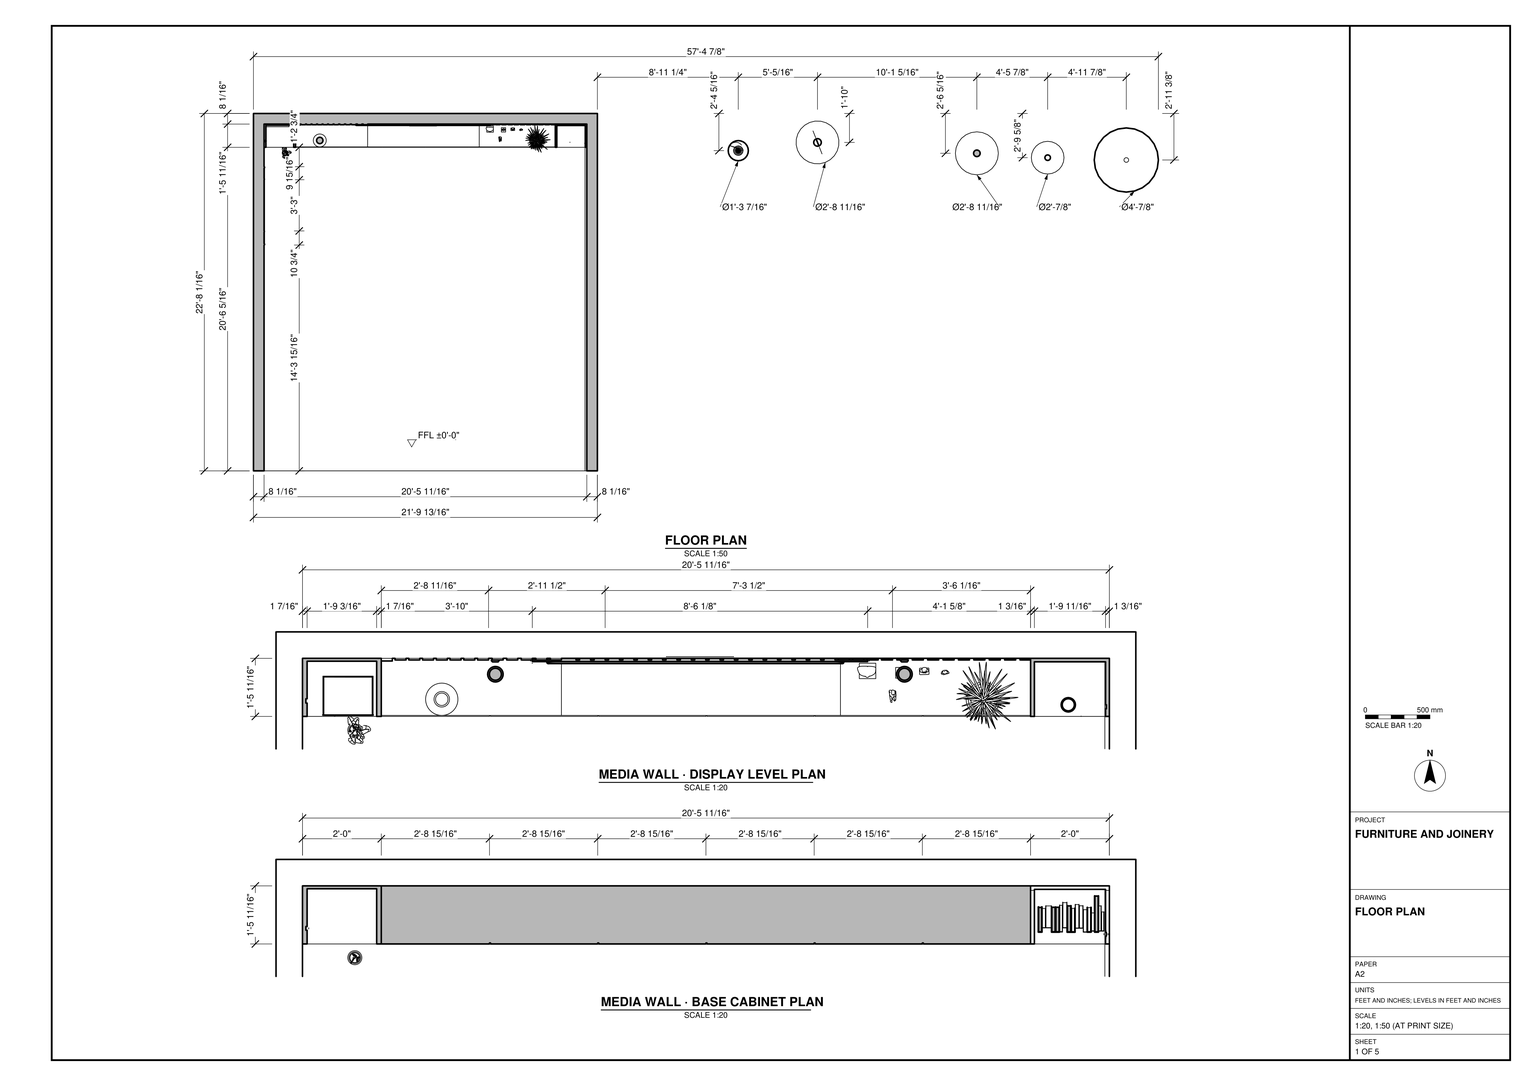
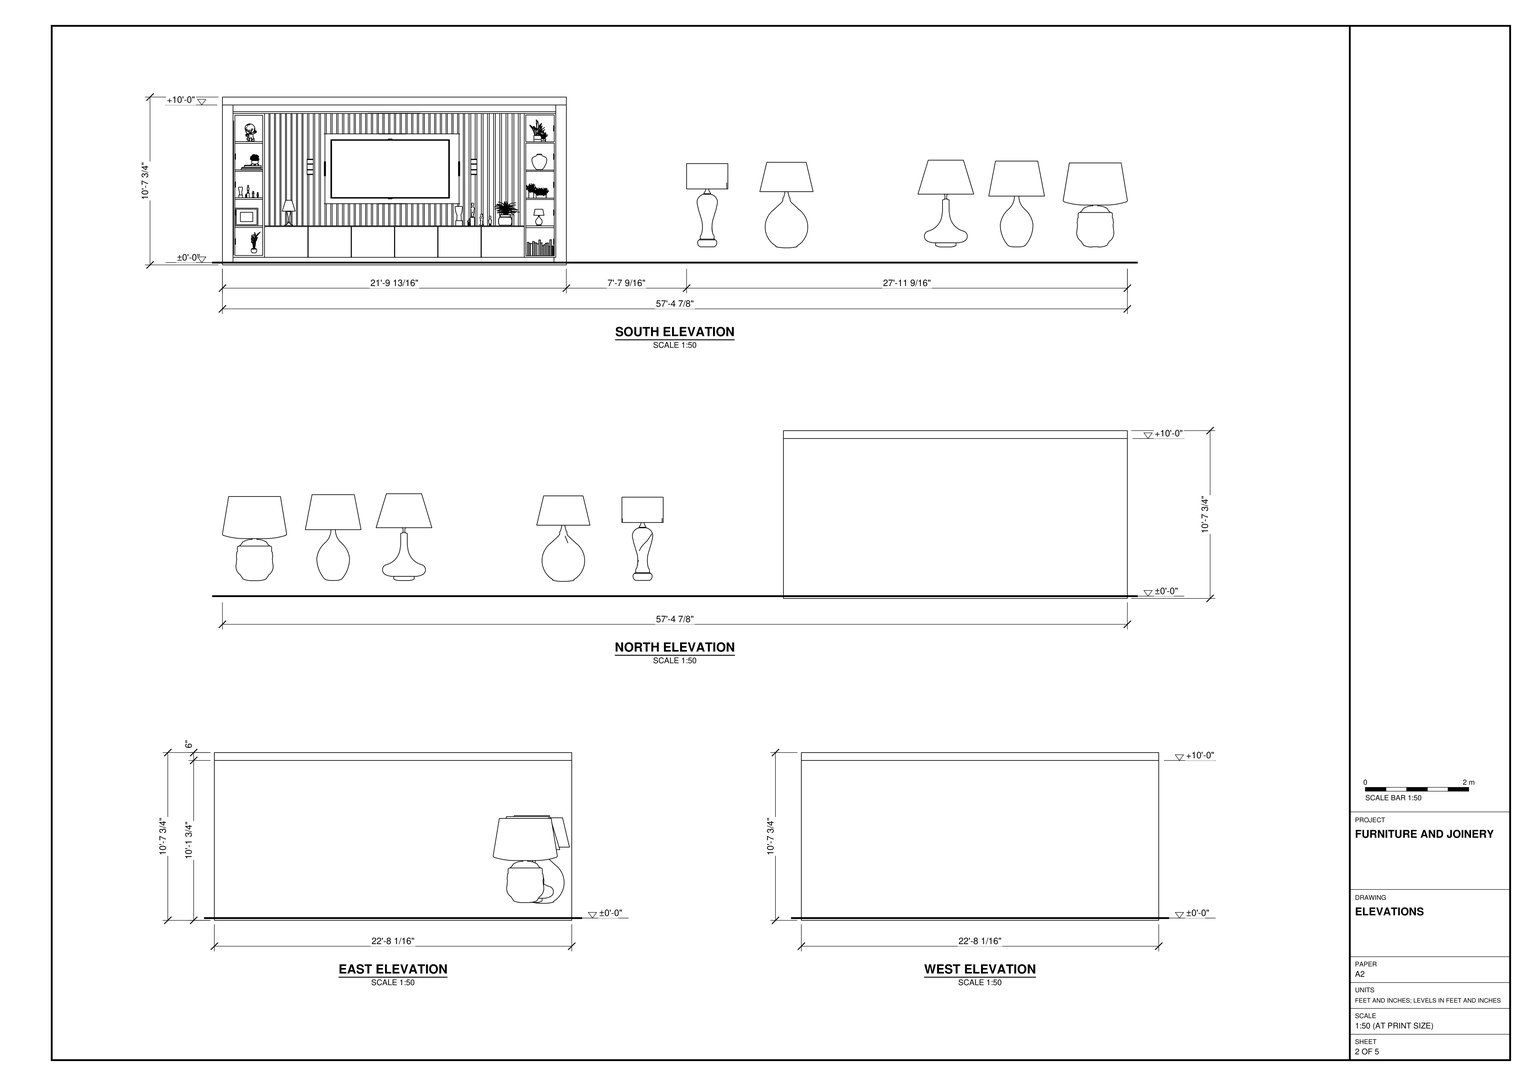
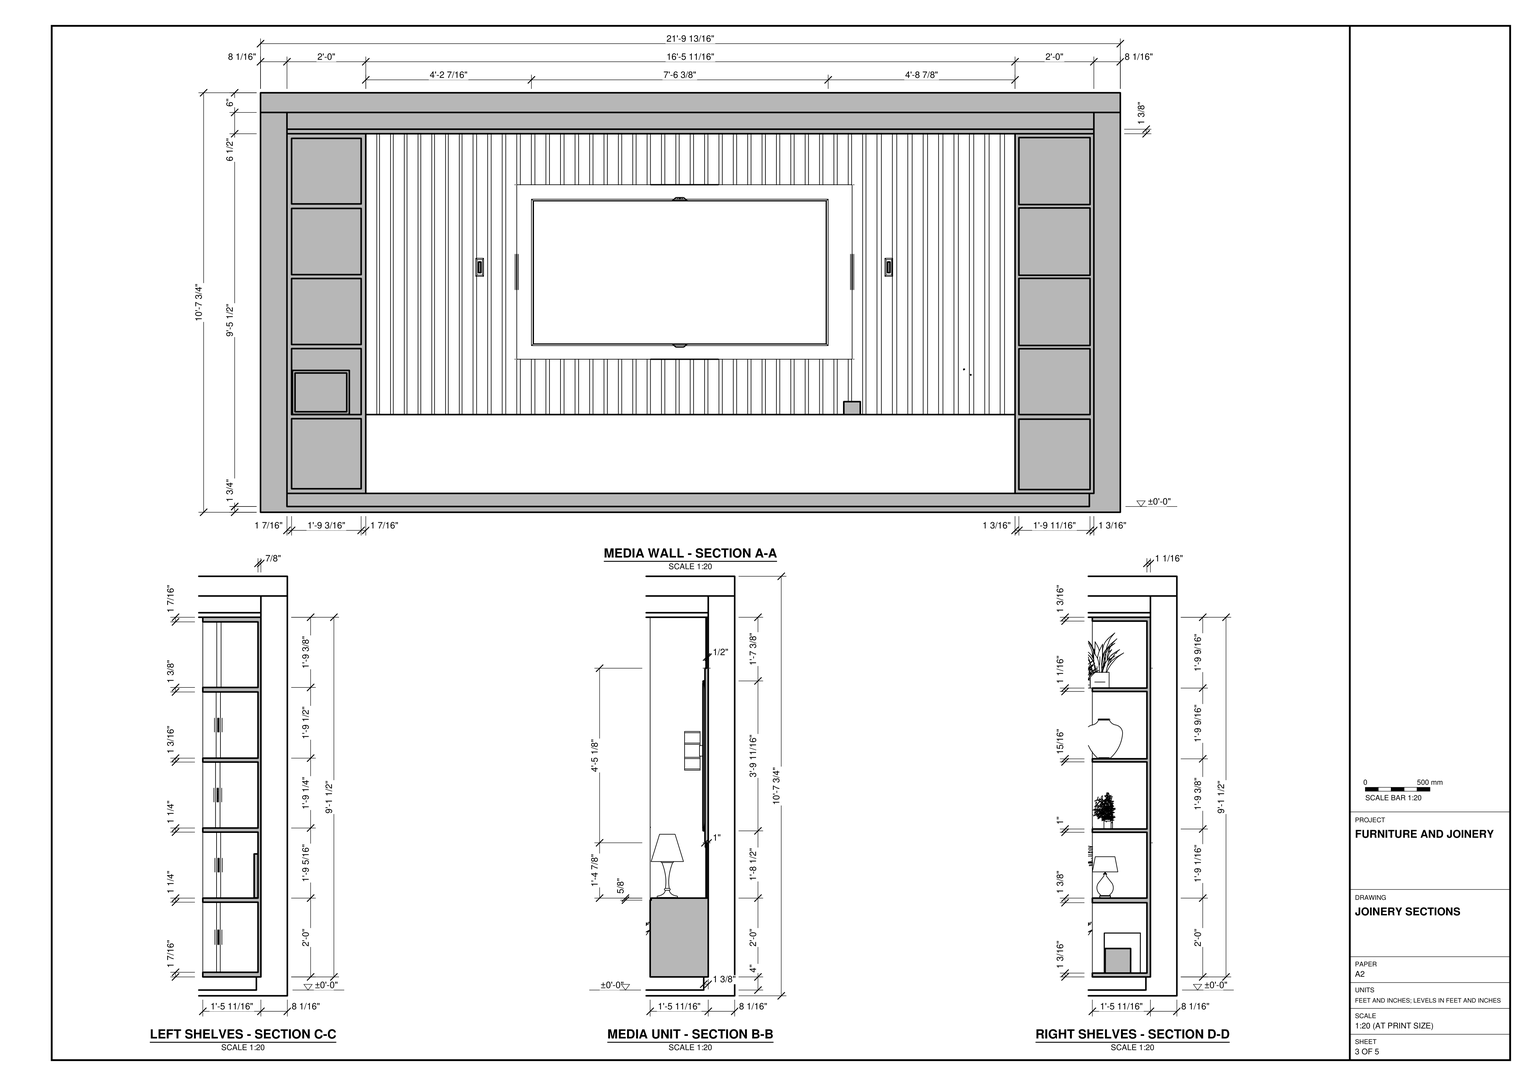
Model the media wall and its three-sided room shell in SketchUp from task_files/diagram_01.pdf. Work in feet and inches, with the finished floor at ±0'-0". Including the freestanding lamps to the right of the shell, the overall model is 57'-4 7/8" wide, 22'-8 1/16" deep and 10'-7 3/4" high. Use the 8 1/16" wall thickness shown in plan. Include the floor slab, upper slab and window unit, and leave the front open as shown in the south elevation.

Fit the joinery across the 20'-5 11/16" clear width of the rear wall. Use the base cabinet plan to divide the low cabinet run into six equal fronts above a recessed plinth. At each end, build a tall open shelving unit with the shelf spacing shown in its section. Between the shelving units, model the vertical slats behind the framed rectangular display. Place the books, plants and small display objects on the shelves and cabinet top. Position the five freestanding lamps as shown in plan, preserving the larger gap between the second and third lamps. Any suitable library components may be used for lamps, plants, books and other loose items.

Keep each shell element and each furniture or joinery piece in a separate group or component, and use components for repeated parts. Save one SketchUp model as output_files/built_in_media_wall_with_flanking_display_shelves.skp.

# SketchUp Ruby script. Lengths in inches.
U = 1.inch
M = Sketchup.active_model
def pt(a) = Geom::Point3d.new(a.map { |v| v * U })
def face(e, loops, mat)
  f = e.add_face(loops[0].map { |a| pt(a) })
  loops[1..].each { |l| e.add_face(l.map { |a| pt(a) }).erase! }
  f.material = f.back_material = mat if mat
  f
end
# faces: each face lists its corners as indices into pts; further lists are holes
def faces(e, pts, list, mat = nil) = list.each { |f| face(e, (f[0].is_a?(Array) ? f : [f]).map { |l| l.map { |i| pts[i] } }, mat) }
# xy, xz, yz: faces in a plane at the given z, y or x. An outline is a flat list of corners, or four numbers for a rectangle; further outlines are holes
def ring(l) = l.size == 4 ? [[l[0], l[1]], [l[2], l[1]], [l[2], l[3]], [l[0], l[3]]] : l.each_slice(2).to_a
def flat(e, list, mat, &to3) = list.each { |f| face(e, (f[0].is_a?(Array) ? f : [f]).map { |l| ring(l).map { |u, v| to3.(u, v) } }, mat) }
def xy(e, z, list, mat = nil) = flat(e, list, mat) { |x, y| [x, y, z] }
def xz(e, y, list, mat = nil) = flat(e, list, mat) { |x, z| [x, y, z] }
def yz(e, x, list, mat = nil) = flat(e, list, mat) { |y, z| [x, y, z] }
def lines(e, pts, list) = list.each { |a, b| e.add_line(pt(pts[a]), pt(pts[b])) }
# prism: a flat outline (further loops are holes) pulled along v
def prism(e, loops, v, mat = nil)
  f = face(e, loops, mat); d = Geom::Vector3d.new(v.map { |x| x * U })
  f.pushpull(f.normal.samedirection?(d) ? d.length : -d.length)
end
def box(e, o, s, mat = nil) = prism(e, [[o, [o[0] + s[0], o[1], o[2]], [o[0] + s[0], o[1] + s[1], o[2]], [o[0], o[1] + s[1], o[2]]]], [0, 0, s[2]], mat)
def at(x, y, z, deg = 0) = Geom::Transformation.translation(pt([x, y, z])) * Geom::Transformation.rotation(ORIGIN, Z_AXIS, deg.degrees)
def axes(o, x, y, z) = Geom::Transformation.new([*x, 0, *y, 0, *z, 0, *pt(o).to_a, 1])
def part(name) = M.definitions.add(name)
# library, detail: a bought-in or finely detailed component or shape, given as its bounding box
def library(name, o, s) = part(name).tap { |d| box(d.entities, o, s) }
def detail(e, o, s) = box(e.add_group.entities, o, s)
def put(e, d, t, mat = nil) = e.add_instance(d, t).tap { |i| i.material = mat if mat }
def group(e, t, mat = nil) = e.add_group.tap { |g| g.transformation = t; g.material = mat if mat }.entities
root = M.entities
M.materials.add("Generic").color = [230, 212, 196]
M.materials.add("[Color C01]").color = [255, 229, 204]
M.materials.add("[Color D01]").color = [168, 159, 134]
M.materials.add("[Color M08]").color = [30, 30, 30]
M.materials.add("[Color_008]").color = [30, 30, 30]
M.materials.add("[Granite Dark Gray]").color = [69, 68, 68]
M.materials.add("[Groundcover_RiverRock_4inch]").color = [145, 126, 109]
c1 = library("Wall+spot",[0,0,0],[4.72,6.7,11.8125])
c2 = library("Flat screen television",[0,1.41,1.14],[35.92,0.28,20.21])
c3 = library("Spot Light",[-5.1,-5.1,-11.05],[10.2,10.2,11.05])
c4 = library("Spot Light\#1",[-5.1,-5.1,-11.05],[10.2,10.2,11.05])
c5 = library("ADORNOS+LIVROS+PLANTA+CELULAR+ÓCULOS",[6.19,-1.3125,-0.22],[15.35,11.9,12.07])
c6 = library("Cycladic+Idols",[-6.2,-43.67,0],[139.39,59.86,86.49])
c7 = part("Picture frame")
xy(c7.entities,0,[[[-0.79,-0.79,16.54,12.6],[0,0,15.75,11.8125]],[[0,0,15.75,11.8125],[3.15,2.36,12.6,9.45]]])
xy(c7.entities,0.79,[[[0,0,15.75,11.8125],[3.15,2.36,12.6,9.45]]])
xy(c7.entities,1.18,[[[-0.79,-0.79,16.54,12.6],[0,0,15.75,11.8125]]],"[Color_008]")
xz(c7.entities,-0.79,[[-0.79,0,16.54,1.18]],"[Color_008]")
xz(c7.entities,0,[[0,0,15.75,0.79]])
xz(c7.entities,0,[[0,0.79,15.75,1.18]],"[Color_008]")
xz(c7.entities,2.36,[[3.15,0,12.6,0.79]])
xz(c7.entities,9.45,[[3.15,0,12.6,0.79]])
xz(c7.entities,11.8125,[[0,0,15.75,0.79]])
xz(c7.entities,11.8125,[[0,0.79,15.75,1.18]],"[Color_008]")
xz(c7.entities,12.6,[[-0.79,0,16.54,1.18]],"[Color_008]")
yz(c7.entities,-0.79,[[-0.79,0,12.6,1.18]],"[Color_008]")
yz(c7.entities,0,[[0,0,11.8125,0.79]])
yz(c7.entities,0,[[0,0.79,11.8125,1.18]],"[Color_008]")
yz(c7.entities,3.15,[[2.36,0,9.45,0.79]])
yz(c7.entities,12.6,[[2.36,0,9.45,0.79]])
yz(c7.entities,15.75,[[0,0,11.8125,0.79]])
yz(c7.entities,15.75,[[0,0.79,11.8125,1.18]],"[Color_008]")
yz(c7.entities,16.54,[[-0.79,0,12.6,1.18]],"[Color_008]")
g1 = group(c7.entities,at(0,0,0.79))
xy(g1,0,[[3.15,2.36,12.6,9.45]],"[Groundcover_RiverRock_4inch]")
c8 = library("Potted broadleaf plant",[-29.7,0,-10.87],[31.67,38.52,72.45])
c9 = library("Potted plant pair",[-0.125,-0.11,0],[4.84,5.4,5.74])
c10 = library("interior plants_leaves_small",[-1.83,-3.05,0],[40.47,20.87,24.79])
c11 = library("Pot+Nice",[-24.73,-24.73,-0.79],[49.46,49.46,53.07])
c12 = library("Architecture and design books\#1",[9.67,-0.02,0],[20.02,11.1,12.25])
c13 = library("Potted+Plant",[38.42,1.35,0],[44.68,49.99,41.74])
c14 = library("lamp",[0,0,0],[9.82,9.84,19.44])
c15 = library("Mesh Light\#5",[-0.5,-0.5,-0.1],[1,1,0.2])
c16 = library("Group\#3",[-0.5,-0.5,0],[1,1.5,53.15])
c17 = library("Group\#4",[-0.5,-0.5,-0.1],[103.125,2,0.2])
c18 = library("Group\#5",[-0.5,-0.5,0],[1,1.5,53.15])
c19 = library("Group\#6",[-0.5,-0.5,-0.1],[103.125,2,0.2])
c20 = library("Group\#9",[-0.5,-0.5,0],[1.375,2.125,21.34])
c21 = library("Group\#10",[-0.5,-0.5,0],[1.375,2.25,20.09])
c22 = library("Group\#11",[-0.5,-0.5,0],[1.375,2.375,20.09])
c23 = library("Group\#13",[-0.5,-0.5,0],[1.375,2.3125,20.15])
c24 = library("Group\#17",[-0.5,-0.5,0],[1.25,2.1875,21.4375])
c25 = library("Group\#18",[-0.5,-0.5,0],[1.25,2,20.04])
c26 = library("Group\#19",[-0.5,-0.5,0],[1.25,2,20.4375])
c27 = library("Group\#21",[-0.5,-0.5,0],[1.25,3.07,41.9375])
c28 = library("Group\#26",[0,0,0],[2.77,2.73,4.26])
c29 = library("Group\#40",[0,0,0],[31.4,31.4,63.39])
c30 = library("Group\#39",[0,0,0],[67.07,67.07,107.62])
c31 = library("Group\#38",[0,0,0],[83.73,83.73,135.9375])
c32 = library("Group\#37",[0,0,0],[48.82,48.82,75.96])
c33 = library("Group\#36",[0,0,0],[51.75,51.75,79.68])
c34 = library("Group\#35",[0,0,0],[64.77,64.77,84.93])
xy(root,0,[[0,0,261.8125,272.0625]])
xy(root,1.75,[[8.05,0,252.38,262.63]],"Generic")
xy(root,5.75,[[252.38,0,253.76,246.32],[8.05,246.32,32.05,262.63],[32.05,246.32,32.05,262.63,229.76,262.63,229.76,246.32,197.11,246.32,197.11,246.62,196.81,246.62,196.81,246.32,164.16,246.32,164.16,246.62,163.86,246.62,163.86,246.32,131.21,246.32,131.21,246.62,130.91,246.62,130.91,246.32,98.26,246.32,98.26,246.62,97.96,246.62,97.96,246.32,65.3,246.32,65.3,246.62,65,246.62,65,246.32],[229.76,246.32,252.38,262.63],[252.38,246.32,253.76,262.63],
  [8.05,262.63,32.05,264.01],[32.05,262.63,229.76,264.01],[229.76,262.63,253.76,264.01]])
xy(root,6.92,[[252.38,246.32,252.59,246.32,252.59,248.7,252.84,248.7,252.84,249.88,252.59,249.88,252.59,262.95,252.38,262.95]])
xy(root,6.92,[[230.93,246.32,252.38,262.95]],"[Color C01]")
xy(root,7.16,[[9.46,246.32,30.64,246.32,30.64,263.13,9.46,263.13,9.46,251.63,9.09,251.63,9.09,250.51,9.46,250.51]],"[Color C01]")
xy(root,28.36,[[252.38,246.32,252.38,262.95,252.59,262.95,252.59,249.88,252.84,249.88,252.84,248.7,252.59,248.7,252.59,246.32]])
xy(root,28.36,[[230.93,246.32,252.38,262.95]],"[Color C01]")
xy(root,28.5,[[9.46,246.32,9.46,250.51,9.09,250.51,9.09,251.63,9.46,251.63,9.46,263.13,30.64,263.13,30.64,246.32]],"[Color C01]")
xy(root,29.125,[[32.05,246.32,65,246.62],[65.3,246.32,97.96,246.62],[98.26,246.32,130.91,246.62],[131.21,246.32,163.86,246.62],[164.16,246.32,196.81,246.62],
  [197.11,246.32,229.76,246.62]])
xy(root,29.75,[[9.46,246.32,30.64,246.32,30.64,263.13,9.46,263.13,9.46,251.76,9.09,251.76,9.09,250.51,9.46,250.51],[252.38,246.32,252.59,246.32,252.59,248.88,252.84,248.88,252.84,249.88,252.59,249.88,252.59,262.95,252.38,262.95],[32.05,263.2,35.4,264.01],[36.24,263.51,39.59,264.01],[40.43,263.51,43.78,264.01],
  [44.62,263.51,47.97,264.01],[48.8,263.51,52.15,264.01],[52.99,263.51,56.34,264.01],[57.18,263.51,60.53,264.01],[61.37,263.51,64.72,264.01],
  [65.8,263.51,69.15,264.01],[70.24,263.51,73.59,264.01],[74.68,263.51,78.03,264.01],[79.12,263.51,82.47,264.01],[83.55,263.51,86.9,264.01],
  [87.99,263.51,91.34,264.01],[92.43,263.51,95.78,264.01],[96.87,263.51,100.22,264.01],[101.24,263.51,104.59,264.01],[105.62,263.51,108.97,264.01],
  [109.99,263.51,113.34,264.01],[114.37,263.51,117.72,264.01],[118.74,263.51,122.09,264.01],[123.12,263.51,126.47,264.01],[127.49,263.51,130.84,264.01],
  [131.87,263.51,135.22,264.01],[136.24,263.51,139.59,264.01],[140.62,263.51,143.97,264.01],[144.99,263.51,148.34,264.01],[149.37,263.51,152.72,264.01],
  [153.74,263.51,157.09,264.01],[158.12,263.51,161.47,264.01],[162.49,263.51,165.84,264.01],[166.87,263.51,170.22,264.01],[171.24,263.51,171.87,264.01],
  [171.87,263.51,174.59,264.01],[175.62,263.51,178.97,264.01],[179.99,263.51,183.34,264.01],[184.37,263.51,187.72,264.01],[189.05,263.51,192.4,264.01],
  [193.74,263.51,197.09,264.01],[198.43,263.51,201.78,264.01],[203.12,263.51,206.47,264.01],[207.8,263.51,211.15,264.01],[212.49,263.51,215.84,264.01],
  [217.18,263.51,220.53,264.01],[221.87,263.51,225.22,264.01],[226.55,263.51,229.76,264.01]])
xy(root,29.75,[[230.93,246.32,252.38,262.95],[32.05,246.62,86.9,246.62,86.9,263.51,83.55,263.51,83.55,264.01,82.47,264.01,82.47,263.51,79.12,263.51,79.12,264.01,78.03,264.01,78.03,263.51,74.68,263.51,74.68,264.01,73.59,264.01,73.59,263.51,70.24,263.51,70.24,264.01,69.15,264.01,69.15,263.51,65.8,263.51,65.8,264.01,64.72,264.01,64.72,263.51,61.37,263.51,61.37,264.01,60.53,264.01,60.53,263.51,57.18,263.51,57.18,264.01,56.34,264.01,56.34,263.51,52.99,263.51,52.99,264.01,52.15,264.01,52.15,263.51,48.8,263.51,48.8,264.01,47.97,264.01,47.97,263.51,44.62,263.51,44.62,264.01,43.78,264.01,43.78,263.51,40.43,263.51,40.43,264.01,39.59,264.01,39.59,263.51,36.24,263.51,36.24,264.01,35.4,264.01,35.4,263.2,32.05,263.2],[171.87,246.62,229.76,246.62,229.76,263.51,226.55,263.51,226.55,264.01,225.22,264.01,225.22,263.51,221.87,263.51,221.87,264.01,220.53,264.01,220.53,263.51,217.18,263.51,217.18,264.01,215.84,264.01,215.84,263.51,212.49,263.51,212.49,264.01,211.15,264.01,211.15,263.51,207.8,263.51,207.8,264.01,206.47,264.01,206.47,263.51,203.12,263.51,203.12,264.01,201.78,264.01,201.78,263.51,198.43,263.51,198.43,264.01,197.09,264.01,197.09,263.51,193.74,263.51,193.74,264.01,192.4,264.01,192.4,263.51,189.05,263.51,189.05,264.01,187.72,264.01,187.72,263.51,184.37,263.51,184.37,264.01,183.34,264.01,183.34,263.51,179.99,263.51,179.99,264.01,178.97,264.01,178.97,263.51,175.62,263.51,175.62,264.01,174.59,264.01,174.59,263.51,171.87,263.51]],"[Color C01]")
xy(root,29.75,[[86.9,246.62,171.87,246.62,171.87,263.51,171.24,263.51,171.24,264.01,170.22,264.01,170.22,263.51,166.87,263.51,166.87,264.01,165.84,264.01,165.84,263.51,162.49,263.51,162.49,264.01,161.47,264.01,161.47,263.51,158.12,263.51,158.12,264.01,157.09,264.01,157.09,263.51,153.74,263.51,153.74,264.01,152.72,264.01,152.72,263.51,149.37,263.51,149.37,264.01,148.34,264.01,148.34,263.51,144.99,263.51,144.99,264.01,143.97,264.01,143.97,263.51,140.62,263.51,140.62,264.01,139.59,264.01,139.59,263.51,136.24,263.51,136.24,264.01,135.22,264.01,135.22,263.51,131.87,263.51,131.87,264.01,130.84,264.01,130.84,263.51,127.49,263.51,127.49,264.01,126.47,264.01,126.47,263.51,123.12,263.51,123.12,264.01,122.09,264.01,122.09,263.51,118.74,263.51,118.74,264.01,117.72,264.01,117.72,263.51,114.37,263.51,114.37,264.01,113.34,264.01,113.34,263.51,109.99,263.51,109.99,264.01,108.97,264.01,108.97,263.51,105.62,263.51,105.62,264.01,104.59,264.01,104.59,263.51,101.24,263.51,101.24,264.01,100.22,264.01,100.22,263.51,96.87,263.51,96.87,264.01,95.78,264.01,95.78,263.51,92.43,263.51,92.43,264.01,91.34,264.01,91.34,263.51,87.99,263.51,87.99,264.01,86.9,264.01]],"[Granite Dark Gray]")
xy(root,49.79,[[252.38,246.32,252.38,262.95,252.59,262.95,252.59,249.88,252.84,249.88,252.84,248.88,252.59,248.88,252.59,246.32]])
xy(root,49.79,[[230.93,246.32,252.38,262.95]],"[Color C01]")
xy(root,49.84,[[9.46,246.32,9.46,250.51,9.09,250.51,9.09,251.76,9.46,251.76,9.46,263.13,30.64,263.13,30.64,246.32]],"[Color C01]")
xy(root,50.79,[[230.93,246.32,252.38,262.95],[252.38,246.32,252.59,246.32,252.59,248.88,252.84,248.88,252.84,249.89,252.59,249.89,252.59,262.95,252.38,262.95]])
xy(root,51.09,[[9.46,246.32,30.64,246.32,30.64,263.13,9.46,263.13,9.46,251.57,9.09,251.57,9.09,250.2,9.46,250.2]])
xy(root,71.18,[[9.46,246.32,9.46,250.2,9.09,250.2,9.09,251.57,9.46,251.57,9.46,263.13,30.64,263.13,30.64,246.32]],"[Color C01]")
xy(root,71.23,[[252.38,246.32,252.38,262.95,252.59,262.95,252.59,249.89,252.84,249.89,252.84,248.88,252.59,248.88,252.59,246.32]])
xy(root,71.23,[[230.93,246.32,252.38,262.95]],"[Color C01]")
xy(root,72.17,[[252.38,246.32,252.59,246.32,252.59,248.64,252.84,248.64,252.84,249.89,252.59,249.89,252.59,262.95,252.38,262.95]])
xy(root,72.17,[[230.93,246.32,252.38,262.95]],"[Color C01]")
xy(root,72.37,[[9.46,246.32,30.64,246.32,30.64,263.13,9.46,263.13,9.46,251.7,9.09,251.7,9.09,250.38,9.46,250.38]])
xy(root,92.52,[[9.46,246.32,9.46,250.38,9.09,250.38,9.09,251.7,9.46,251.7,9.46,263.13,30.64,263.13,30.64,246.32]],"[Color C01]")
xy(root,92.67,[[230.93,246.32,230.93,262.95,252.59,262.95,252.59,249.89,252.84,249.89,252.84,248.64,252.59,248.64,252.59,246.32]],"[Color C01]")
xy(root,93.71,[[230.93,246.32,252.59,246.32,252.59,249.14,252.84,249.14,252.84,250.71,252.59,250.71,252.59,262.95,230.93,262.95]],"[Color C01]")
xy(root,93.9,[[9.46,246.32,30.64,246.32,30.64,263.13,9.46,263.13,9.46,251.88,9.09,251.88,9.09,250.57,9.46,250.57]])
xy(root,113.87,[[9.46,246.32,9.46,250.57,9.09,250.57,9.09,251.88,9.46,251.88,9.46,263.13,30.64,263.13,30.64,246.32]],"[Color C01]")
xy(root,114.11,[[252.38,246.32,252.38,262.95,252.59,262.95,252.59,250.71,252.84,250.71,252.84,249.14,252.59,249.14,252.59,246.32]])
xy(root,114.11,[[230.93,246.32,252.38,262.95]],"[Color C01]")
xy(root,115.28,[[8.05,246.32,32.05,264.01],[229.76,246.32,253.76,264.01],[32.05,263.2,35.4,264.01],[36.24,263.51,39.59,264.01],[40.43,263.51,43.78,264.01],
  [44.62,263.51,47.97,264.01],[48.8,263.51,52.15,264.01],[52.99,263.51,56.34,264.01],[57.18,263.51,60.53,264.01],[61.37,263.51,64.72,264.01],
  [65.8,263.51,69.15,264.01],[70.24,263.51,73.59,264.01],[74.68,263.51,78.03,264.01],[79.12,263.51,82.47,264.01],[83.55,263.51,86.9,264.01],
  [87.99,263.51,91.34,264.01],[92.43,263.51,95.78,264.01],[96.87,263.51,100.22,264.01],[101.24,263.51,104.59,264.01],[105.62,263.51,108.97,264.01],
  [109.99,263.51,113.34,264.01],[114.37,263.51,117.72,264.01],[118.74,263.51,122.09,264.01],[123.12,263.51,126.47,264.01],[127.49,263.51,130.84,264.01],
  [131.87,263.51,135.22,264.01],[136.24,263.51,139.59,264.01],[140.62,263.51,143.97,264.01],[144.99,263.51,148.34,264.01],[149.37,263.51,152.72,264.01],
  [153.74,263.51,157.09,264.01],[158.12,263.51,161.47,264.01],[162.49,263.51,165.84,264.01],[166.87,263.51,170.22,264.01],[171.24,263.51,174.59,264.01],
  [175.62,263.51,178.97,264.01],[179.99,263.51,183.34,264.01],[184.37,263.51,187.72,264.01],[189.05,263.51,192.4,264.01],[193.74,263.51,197.09,264.01],
  [198.43,263.51,201.78,264.01],[203.12,263.51,206.47,264.01],[207.8,263.51,211.15,264.01],[212.49,263.51,215.84,264.01],[217.18,263.51,220.53,264.01],
  [221.87,263.51,225.22,264.01],[226.55,263.51,229.76,264.01]])
xy(root,121.75,[[0,0,0,272.0625,261.8125,272.0625,261.8125,0,253.76,0,253.76,264.01,8.05,264.01,8.05,0],[8.05,0,253.76,264.01]])
xy(root,127.75,[[0,0,261.8125,272.0625]])
xz(root,0,[[0,0,261.8125,0,261.8125,121.75,253.76,121.75,253.76,5.75,252.38,5.75,252.38,1.75,8.05,1.75,8.05,121.75,0,121.75],[0,121.75,261.8125,127.75]])
xz(root,246.32,[[32.05,5.75,65,29.125],[65.3,5.75,97.96,29.125],[98.26,5.75,130.91,29.125],[131.21,5.75,163.86,29.125],[164.16,5.75,196.81,29.125],
  [197.11,5.75,229.76,29.125]],"[Color C01]")
xz(root,246.32,[[[8.05,5.75,32.05,115.28],[9.46,7.16,30.64,113.87]],[[229.76,5.75,253.76,115.28],[230.93,6.92,252.59,92.67],[230.93,93.71,252.59,114.11]],[230.93,28.36,252.59,29.75],[9.46,28.5,30.64,29.75],[230.93,49.79,252.59,50.79],
  [9.46,49.84,30.64,51.09],[9.46,71.18,30.64,72.37],[230.93,71.23,252.59,72.17],[9.46,92.52,30.64,93.9]],"[Color M08]")
xz(root,246.62,[[65,5.75,65.3,29.125],[97.96,5.75,98.26,29.125],[130.91,5.75,131.21,29.125],[163.86,5.75,164.16,29.125],[196.81,5.75,197.11,29.125],
  [32.05,29.125,229.76,29.75]])
xz(root,248.64,[[252.59,72.17,252.84,92.21],[252.59,92.21,252.84,92.67]])
xz(root,248.7,[[252.59,6.92,252.84,28.36]])
xz(root,248.88,[[252.59,29.75,252.84,49.79],[252.59,50.79,252.84,70.84],[252.59,70.84,252.84,71.23]])
xz(root,249.14,[[252.59,93.71,252.84,94.32],[252.59,94.32,252.84,114.11]])
xz(root,249.89,[[252.59,70.84,252.84,71.23],[252.59,92.21,252.84,92.67]])
xz(root,250.2,[[9.09,51.09,9.46,71.18]])
xz(root,250.38,[[9.09,72.37,9.46,92.52]])
xz(root,250.51,[[9.09,7.16,9.46,28.5],[9.09,29.75,9.46,49.84]])
xz(root,250.57,[[9.09,93.9,9.46,113.87]])
xz(root,262.63,[[8.05,1.75,252.38,5.75]],"[Color C01]")
xz(root,262.95,[[230.93,6.92,252.59,28.36],[230.93,29.75,252.59,49.79],[230.93,50.79,252.59,71.23],[230.93,72.17,252.59,92.67],[230.93,93.71,252.59,114.11]],"[Color C01]")
xz(root,263.01,[[78.03,46.6,180.15,99.75]],"[Color C01]")
xz(root,263.13,[[9.46,7.16,30.64,28.5],[9.46,29.75,30.64,49.84],[9.46,51.09,30.64,71.18],[9.46,72.37,30.64,92.52],[9.46,93.9,30.64,113.87]],"[Color C01]")
xz(root,263.2,[[32.05,29.75,35.4,115.28]],"[Color C01]")
xz(root,263.51,[[78.03,46.6,79.12,99.75],[79.12,46.6,82.47,99.75],[82.47,46.6,83.55,99.75],[83.55,46.6,86.9,99.75],[91.34,46.6,92.43,99.75],
  [95.78,46.6,96.87,99.75],[100.22,46.6,101.24,99.75],[104.59,46.6,105.62,99.75],[108.97,46.6,109.99,99.75],[113.34,46.6,114.37,99.75],
  [117.72,46.6,118.74,99.75],[122.09,46.6,123.12,99.75],[126.47,46.6,127.49,99.75],[130.84,46.6,131.87,99.75],[135.22,46.6,136.24,99.75],
  [139.59,46.6,140.62,99.75],[143.97,46.6,144.99,99.75],[148.34,46.6,149.37,99.75],[152.72,46.6,153.74,99.75],[157.09,46.6,158.12,99.75],
  [161.47,46.6,162.49,99.75],[165.84,46.6,166.87,99.75],[170.22,46.6,171.24,99.75],[171.24,46.6,174.59,99.75],[174.59,46.6,175.62,99.75],
  [175.62,46.6,178.97,99.75],[178.97,46.6,179.99,99.75],[179.99,46.6,180.15,99.75]])
xz(root,263.51,[[36.24,29.75,39.59,115.28],[40.43,29.75,43.78,115.28],[44.62,29.75,47.97,115.28],[48.8,29.75,52.15,115.28],[52.99,29.75,56.34,115.28],
  [57.18,29.75,60.53,115.28],[61.37,29.75,64.72,115.28],[65.8,29.75,69.15,115.28],[70.24,29.75,73.59,115.28],[74.68,29.75,78.03,115.28],
  [79.12,29.75,82.47,46.6],[83.55,29.75,86.9,46.6],[87.99,29.75,91.34,46.6],[92.43,29.75,95.78,46.6],[96.87,29.75,100.22,46.6],
  [101.24,29.75,104.59,46.6],[105.62,29.75,108.97,46.6],[109.99,29.75,113.34,46.6],[114.37,29.75,117.72,46.6],[118.74,29.75,122.09,46.6],
  [123.12,29.75,126.47,46.6],[127.49,29.75,130.84,46.6],[131.87,29.75,135.22,46.6],[136.24,29.75,139.59,46.6],[140.62,29.75,143.97,46.6],
  [144.99,29.75,148.34,46.6],[149.37,29.75,152.72,46.6],[153.74,29.75,157.09,46.6],[158.12,29.75,161.47,46.6],[162.49,29.75,165.84,46.6],
  [166.87,29.75,170.22,46.6],[171.24,29.75,174.59,46.6],[175.62,29.75,178.97,46.6],[179.99,29.75,183.34,29.75,183.34,115.28,179.99,115.28,179.99,99.75,180.15,99.75,180.15,46.6,179.99,46.6],[184.37,29.75,187.72,115.28],
  [189.05,29.75,192.4,115.28],[193.74,29.75,197.09,115.28],[198.43,29.75,201.78,115.28],[203.12,29.75,206.47,115.28],[207.8,29.75,211.15,115.28],
  [212.49,29.75,215.84,115.28],[217.18,29.75,220.53,115.28],[221.87,29.75,225.22,115.28],[226.55,29.75,229.76,115.28],[79.12,99.75,82.47,115.28],
  [83.55,99.75,86.9,115.28],[87.99,99.75,91.34,115.28],[92.43,99.75,95.78,115.28],[96.87,99.75,100.22,115.28],[101.24,99.75,104.59,115.28],
  [105.62,99.75,108.97,115.28],[109.99,99.75,113.34,115.28],[114.37,99.75,117.72,115.28],[118.74,99.75,122.09,115.28],[123.12,99.75,126.47,115.28],
  [127.49,99.75,130.84,115.28],[131.87,99.75,135.22,115.28],[136.24,99.75,139.59,115.28],[140.62,99.75,143.97,115.28],[144.99,99.75,148.34,115.28],
  [149.37,99.75,152.72,115.28],[153.74,99.75,157.09,115.28],[158.12,99.75,161.47,115.28],[162.49,99.75,165.84,115.28],[166.87,99.75,170.22,115.28],
  [171.24,99.75,174.59,115.28],[175.62,99.75,178.97,115.28]],"[Color C01]")
xz(root,264.01,[[8.05,5.75,32.05,115.28],[32.05,5.75,229.76,29.75],[229.76,5.75,229.76,29.75,229.9,29.75,229.9,115.28,253.76,115.28,253.76,5.75],[86.9,29.75,87.99,46.6],[87.99,29.75,91.34,115.28],
  [92.43,29.75,95.78,115.28],[96.87,29.75,100.22,115.28],[101.24,29.75,104.59,115.28],[105.62,29.75,108.97,115.28],[109.99,29.75,113.34,115.28],
  [114.37,29.75,117.72,115.28],[118.74,29.75,122.09,115.28],[123.12,29.75,126.47,115.28],[127.49,29.75,130.84,115.28],[131.87,29.75,135.22,115.28],
  [136.24,29.75,139.59,115.28],[140.62,29.75,143.97,115.28],[144.99,29.75,148.34,115.28],[149.37,29.75,152.72,115.28],[153.74,29.75,157.09,115.28],
  [158.12,29.75,161.47,115.28],[162.49,29.75,165.84,115.28],[166.87,29.75,170.22,115.28],[171.24,29.75,174.59,115.28],[175.62,29.75,178.97,115.28],
  [179.99,29.75,183.34,115.28],[184.37,29.75,187.72,115.28],[189.05,29.75,192.4,115.28],[193.74,29.75,197.09,115.28],[198.43,29.75,201.78,115.28],
  [203.12,29.75,206.47,115.28],[207.8,29.75,211.15,115.28],[212.49,29.75,215.84,115.28],[217.18,29.75,220.53,115.28],[221.87,29.75,225.22,115.28],
  [226.55,29.75,229.76,115.28],[229.76,29.75,229.9,115.28],[86.9,46.6,87.99,99.75]])
xz(root,264.01,[[35.4,29.75,36.24,29.75,36.24,115.28,39.59,115.28,39.59,29.75,40.43,29.75,40.43,115.28,43.78,115.28,43.78,29.75,44.62,29.75,44.62,115.28,47.97,115.28,47.97,29.75,48.8,29.75,48.8,115.28,52.15,115.28,52.15,29.75,52.99,29.75,52.99,115.28,56.34,115.28,56.34,29.75,57.18,29.75,57.18,115.28,60.53,115.28,60.53,29.75,61.37,29.75,61.37,115.28,64.72,115.28,64.72,29.75,65.8,29.75,65.8,115.28,69.15,115.28,69.15,29.75,70.24,29.75,70.24,115.28,73.59,115.28,73.59,29.75,74.68,29.75,74.68,115.28,78.03,115.28,78.03,29.75,79.12,29.75,79.12,115.28,82.47,115.28,82.47,29.75,83.55,29.75,83.55,115.28,86.9,115.28,86.9,99.75,87.99,99.75,87.99,115.28,91.34,115.28,91.34,29.75,92.43,29.75,92.43,115.28,95.78,115.28,95.78,29.75,96.87,29.75,96.87,115.28,100.22,115.28,100.22,29.75,101.24,29.75,101.24,115.28,104.59,115.28,104.59,29.75,105.62,29.75,105.62,115.28,108.97,115.28,108.97,29.75,109.99,29.75,109.99,115.28,113.34,115.28,113.34,29.75,114.37,29.75,114.37,115.28,117.72,115.28,117.72,29.75,118.74,29.75,118.74,115.28,122.09,115.28,122.09,29.75,123.12,29.75,123.12,115.28,126.47,115.28,126.47,29.75,127.49,29.75,127.49,115.28,130.84,115.28,130.84,29.75,131.87,29.75,131.87,115.28,135.22,115.28,135.22,29.75,136.24,29.75,136.24,115.28,139.59,115.28,139.59,29.75,140.62,29.75,140.62,115.28,143.97,115.28,143.97,29.75,144.99,29.75,144.99,115.28,148.34,115.28,148.34,29.75,149.37,29.75,149.37,115.28,152.72,115.28,152.72,29.75,153.74,29.75,153.74,115.28,157.09,115.28,157.09,29.75,158.12,29.75,158.12,115.28,161.47,115.28,161.47,29.75,162.49,29.75,162.49,115.28,165.84,115.28,165.84,29.75,166.87,29.75,166.87,115.28,170.22,115.28,170.22,29.75,171.24,29.75,171.24,115.28,174.59,115.28,174.59,29.75,175.62,29.75,175.62,115.28,178.97,115.28,178.97,29.75,179.99,29.75,179.99,115.28,183.34,115.28,183.34,29.75,184.37,29.75,184.37,115.28,187.72,115.28,187.72,29.75,189.05,29.75,189.05,115.28,192.4,115.28,192.4,29.75,193.74,29.75,193.74,115.28,197.09,115.28,197.09,29.75,198.43,29.75,198.43,115.28,201.78,115.28,201.78,29.75,203.12,29.75,203.12,115.28,206.47,115.28,206.47,29.75,207.8,29.75,207.8,115.28,211.15,115.28,211.15,29.75,212.49,29.75,212.49,115.28,215.84,115.28,215.84,29.75,217.18,29.75,217.18,115.28,220.53,115.28,220.53,29.75,221.87,29.75,221.87,115.28,225.22,115.28,225.22,29.75,226.55,29.75,226.55,115.28,253.76,115.28,253.76,121.75,8.05,121.75,8.05,115.28,35.4,115.28]],"[Color D01]")
xz(root,272.0625,[[0,0,261.8125,121.75],[0,121.75,261.8125,127.75]])
yz(root,0,[[0,0,272.0625,121.75],[0,121.75,272.0625,127.75]])
yz(root,8.05,[[246.32,5.75,264.01,115.28],[95.52,7.93,154.08,109.31]])
yz(root,8.05,[[[0,1.75,262.63,1.75,262.63,5.75,246.32,5.75,246.32,115.28,264.01,115.28,264.01,121.75,0,121.75],[171.9,7.37,171.9,109.87,231.58,109.87,231.58,7.93,230.77,7.93,230.77,7.37],[95.52,7.93,154.08,109.31]],[[172.96,8.43,230.52,108.81],[181.86,11.98,181.86,102.29,222.42,102.29,222.42,12.35,221.61,12.35,221.61,11.98]],[182.67,12.79,221.61,101.48]],"[Color C01]")
yz(root,8.3,[[182.18,12.3,182.27,12.38,182.27,101.88,182.18,101.97],[182.18,12.3,221.48,12.3,221.47,12.38,182.27,12.38],[221.93,12.35,222.02,12.35,222.02,101.88,221.93,101.8],[222.02,12.35,222.1,12.35,222.1,101.97,222.02,101.88],[182.27,12.38,182.35,12.47,182.35,101.8,182.27,101.88],
  [182.27,12.38,221.47,12.38,221.48,12.47,182.35,12.47],[182.35,101.8,221.93,101.8,222.02,101.88,182.27,101.88],[182.27,101.88,222.02,101.88,222.1,101.97,182.18,101.97]],"[Color C01]")
yz(root,9.46,[[246.32,7.16,250.51,28.5],[251.63,7.16,263.13,28.5],[246.32,29.75,250.51,49.84],[251.76,29.75,263.13,49.84],[246.32,51.09,250.2,71.18],
  [251.57,51.09,263.13,71.18],[246.32,72.37,250.38,92.52],[251.7,72.37,263.13,92.52],[246.32,93.9,250.57,113.87],[251.88,93.9,263.13,113.87]],"[Color C01]")
yz(root,30.64,[[246.32,7.16,263.13,28.5],[246.32,29.75,263.13,49.84],[246.32,51.09,263.13,71.18],[246.32,72.37,263.13,92.52],[246.32,93.9,263.13,113.87]])
yz(root,32.05,[[246.32,5.75,264.01,5.75,264.01,29.75,246.62,29.75,246.62,29.125,246.32,29.125],[246.32,29.125,246.62,29.75],[263.2,29.75,264.01,115.28]])
yz(root,32.05,[[246.32,29.75,263.2,115.28]],"[Color C01]")
yz(root,35.4,[[263.2,29.75,264.01,115.28]])
yz(root,36.24,[[263.51,29.75,264.01,115.28]])
yz(root,39.59,[[263.51,29.75,264.01,115.28]])
yz(root,40.43,[[263.51,29.75,264.01,115.28]])
yz(root,43.78,[[263.51,29.75,264.01,115.28]])
yz(root,44.62,[[263.51,29.75,264.01,115.28]])
yz(root,47.97,[[263.51,29.75,264.01,115.28]])
yz(root,48.8,[[263.51,29.75,264.01,115.28]])
yz(root,52.15,[[263.51,29.75,264.01,115.28]])
yz(root,52.99,[[263.51,29.75,264.01,115.28]])
yz(root,56.34,[[263.51,29.75,264.01,115.28]])
yz(root,57.18,[[263.51,29.75,264.01,115.28]])
yz(root,60.53,[[263.51,29.75,264.01,115.28]])
yz(root,61.37,[[263.51,29.75,264.01,115.28]])
yz(root,64.72,[[263.51,29.75,264.01,115.28]])
yz(root,65,[[246.32,5.75,246.62,29.125]])
yz(root,65.3,[[246.32,5.75,246.62,29.125]])
yz(root,65.8,[[263.51,29.75,264.01,115.28]])
yz(root,69.15,[[263.51,29.75,264.01,115.28]])
yz(root,70.24,[[263.51,29.75,264.01,115.28]])
yz(root,73.59,[[263.51,29.75,264.01,115.28]])
yz(root,74.68,[[263.51,29.75,264.01,115.28]])
yz(root,78.03,[[263.51,29.75,264.01,115.28]])
yz(root,79.12,[[263.51,29.75,264.01,115.28]])
yz(root,82.47,[[263.51,29.75,264.01,115.28]])
yz(root,83.55,[[263.51,29.75,264.01,115.28]])
yz(root,86.9,[[263.51,29.75,264.01,46.6],[263.51,46.6,264.01,99.75],[263.51,99.75,264.01,115.28]])
yz(root,87.99,[[263.51,29.75,264.01,46.6],[263.51,99.75,264.01,115.28]])
yz(root,91.34,[[263.51,29.75,264.01,115.28]])
yz(root,92.43,[[263.51,29.75,264.01,115.28]])
yz(root,95.78,[[263.51,29.75,264.01,115.28]])
yz(root,96.87,[[263.51,29.75,264.01,115.28]])
yz(root,97.96,[[246.32,5.75,246.62,29.125]])
yz(root,98.26,[[246.32,5.75,246.62,29.125]])
yz(root,100.22,[[263.51,29.75,264.01,115.28]])
yz(root,101.24,[[263.51,29.75,264.01,115.28]])
yz(root,104.59,[[263.51,29.75,264.01,115.28]])
yz(root,105.62,[[263.51,29.75,264.01,115.28]])
yz(root,108.97,[[263.51,29.75,264.01,115.28]])
yz(root,109.99,[[263.51,29.75,264.01,115.28]])
yz(root,113.34,[[263.51,29.75,264.01,115.28]])
yz(root,114.37,[[263.51,29.75,264.01,115.28]])
yz(root,117.72,[[263.51,29.75,264.01,115.28]])
yz(root,118.74,[[263.51,29.75,264.01,115.28]])
yz(root,122.09,[[263.51,29.75,264.01,115.28]])
yz(root,123.12,[[263.51,29.75,264.01,115.28]])
yz(root,126.47,[[263.51,29.75,264.01,115.28]])
yz(root,127.49,[[263.51,29.75,264.01,115.28]])
yz(root,130.84,[[263.51,29.75,264.01,115.28]])
yz(root,130.91,[[246.32,5.75,246.62,29.125]])
yz(root,131.21,[[246.32,5.75,246.62,29.125]])
yz(root,131.87,[[263.51,29.75,264.01,115.28]])
yz(root,135.22,[[263.51,29.75,264.01,115.28]])
yz(root,136.24,[[263.51,29.75,264.01,115.28]])
yz(root,139.59,[[263.51,29.75,264.01,115.28]])
yz(root,140.62,[[263.51,29.75,264.01,115.28]])
yz(root,143.97,[[263.51,29.75,264.01,115.28]])
yz(root,144.99,[[263.51,29.75,264.01,115.28]])
yz(root,148.34,[[263.51,29.75,264.01,115.28]])
yz(root,149.37,[[263.51,29.75,264.01,115.28]])
yz(root,152.72,[[263.51,29.75,264.01,115.28]])
yz(root,153.74,[[263.51,29.75,264.01,115.28]])
yz(root,157.09,[[263.51,29.75,264.01,115.28]])
yz(root,158.12,[[263.51,29.75,264.01,115.28]])
yz(root,161.47,[[263.51,29.75,264.01,115.28]])
yz(root,162.49,[[263.51,29.75,264.01,115.28]])
yz(root,163.86,[[246.32,5.75,246.62,29.125]])
yz(root,164.16,[[246.32,5.75,246.62,29.125]])
yz(root,165.84,[[263.51,29.75,264.01,115.28]])
yz(root,166.87,[[263.51,29.75,264.01,115.28]])
yz(root,170.22,[[263.51,29.75,264.01,115.28]])
yz(root,171.24,[[263.51,29.75,264.01,115.28]])
yz(root,174.59,[[263.51,29.75,264.01,115.28]])
yz(root,175.62,[[263.51,29.75,264.01,115.28]])
yz(root,178.97,[[263.51,29.75,264.01,115.28]])
yz(root,179.99,[[263.51,29.75,264.01,115.28]])
yz(root,183.34,[[263.51,29.75,264.01,115.28]])
yz(root,184.37,[[263.51,29.75,264.01,115.28]])
yz(root,187.72,[[263.51,29.75,264.01,115.28]])
yz(root,189.05,[[263.51,29.75,264.01,115.28]])
yz(root,192.4,[[263.51,29.75,264.01,115.28]])
yz(root,193.74,[[263.51,29.75,264.01,115.28]])
yz(root,196.81,[[246.32,5.75,246.62,29.125]])
yz(root,197.09,[[263.51,29.75,264.01,115.28]])
yz(root,197.11,[[246.32,5.75,246.62,29.125]])
yz(root,198.43,[[263.51,29.75,264.01,115.28]])
yz(root,201.78,[[263.51,29.75,264.01,115.28]])
yz(root,203.12,[[263.51,29.75,264.01,115.28]])
yz(root,206.47,[[263.51,29.75,264.01,115.28]])
yz(root,207.8,[[263.51,29.75,264.01,115.28]])
yz(root,211.15,[[263.51,29.75,264.01,115.28]])
yz(root,212.49,[[263.51,29.75,264.01,115.28]])
yz(root,215.84,[[263.51,29.75,264.01,115.28]])
yz(root,217.18,[[263.51,29.75,264.01,115.28]])
yz(root,220.53,[[263.51,29.75,264.01,115.28]])
yz(root,221.87,[[263.51,29.75,264.01,115.28]])
yz(root,225.22,[[263.51,29.75,264.01,115.28]])
yz(root,226.55,[[263.51,29.75,264.01,115.28]])
yz(root,229.76,[[246.32,5.75,246.32,29.125,246.62,29.125,246.62,29.75,264.01,29.75,264.01,5.75],[246.32,29.125,246.62,29.75],[263.51,29.75,264.01,115.28]])
yz(root,229.76,[[246.32,29.75,263.51,115.28]],"[Color C01]")
yz(root,230.93,[[246.32,6.92,262.95,28.36],[246.32,29.75,262.95,49.79],[246.32,50.79,262.95,71.23],[246.32,72.17,262.95,92.67],[246.32,93.71,262.95,114.11]],"[Color C01]")
yz(root,252.38,[[0,1.75,262.63,5.75]],"[Color C01]")
yz(root,252.59,[[246.32,6.92,248.7,28.36],[249.88,6.92,262.95,28.36],[246.32,29.75,248.88,49.79],[249.88,29.75,262.95,49.79],[246.32,50.79,248.88,71.23],
  [249.89,50.79,262.95,71.23],[246.32,72.17,248.64,92.67],[249.89,72.17,262.95,92.67],[246.32,93.71,249.14,114.11],[250.71,93.71,262.95,114.11]],"[Color C01]")
yz(root,253.76,[[246.32,5.75,264.01,115.28]])
yz(root,253.76,[[0,5.75,0,121.75,264.01,121.75,264.01,115.28,246.32,115.28,246.32,5.75]],"[Color C01]")
yz(root,261.8125,[[0,0,272.0625,121.75],[0,121.75,272.0625,127.75]])
p = [[8.17,171.9375,109.83],[8.05,171.9,109.87],[8.05,171.9,7.37],[8.17,171.9375,7.41],[8.05,230.52,7.37],[8.05,230.77,7.37],
  [8.17,230.77,7.41],[8.17,230.52,7.41],[8.27,172,109.76],[8.27,172,7.47],[8.27,230.77,7.47],[8.27,230.52,7.47],
  [8.36,172.09,109.68],[8.36,172.09,7.5625],[8.36,230.77,7.5625],[8.36,230.52,7.5625],[8.42,172.19,109.57],[8.42,172.19,7.66],
  [8.42,230.77,7.66],[8.42,230.52,7.66],[8.46,172.31,109.46],[8.46,172.31,7.78],[8.46,230.77,7.78],[8.46,230.52,7.78],
  [8.48,172.43,109.34],[8.48,172.43,7.9],[8.48,230.77,7.9],[8.48,230.52,7.9],[8.46,172.55,109.22],[8.46,172.55,8.02],
  [8.46,230.77,8.02],[8.46,230.52,8.02],[8.05,230.52,7.93],[8.17,230.5625,7.93],[8.17,230.5625,8.39],[8.17,230.5625,108.85],
  [8.05,230.52,108.81],[8.05,230.52,8.43],[8.27,230.63,7.93],[8.27,230.63,8.33],[8.27,230.63,108.91],[8.36,230.71,7.93],
  [8.36,230.71,8.24],[8.36,230.71,109],[8.42,230.82,7.93],[8.42,230.82,109.1],[8.46,230.93,7.93],[8.46,230.93,109.22],
  [8.48,231.05,7.93],[8.48,231.05,109.34],[8.46,231.17,7.93],[8.46,231.17,109.46],[8.42,231.29,7.93],[8.42,231.29,109.57],
  [8.36,231.39,7.93],[8.36,231.39,109.68],[8.27,231.48,7.93],[8.27,231.48,109.76],[8.17,231.54,7.93],[8.05,231.58,7.93],
  [8.05,231.58,109.87],[8.17,231.54,109.83],[8.42,172.66,109.1],[8.42,172.66,8.14],[8.42,230.77,8.14],[8.42,230.52,8.14],
  [8.36,172.77,109],[8.36,172.77,8.24],[8.36,230.77,8.24],[8.36,230.52,8.24],[8.27,172.85,108.91],[8.27,172.85,8.33],
  [8.27,230.77,8.33],[8.27,230.52,8.33],[8.17,172.92,108.85],[8.17,172.92,8.39],[8.17,230.77,8.39],[8.17,230.52,8.39],
  [8.05,172.96,108.81],[8.05,172.96,8.43],[8.05,230.77,8.43],[8.1875,181.96,102.1875],[8.125,181.91,102.24],[8.125,181.91,12.02],
  [8.1875,181.96,12.08],[8.05,181.86,102.29],[8.05,181.86,11.98],[8.125,221.57,12.02],[8.1875,221.54,12.08],[8.05,221.61,11.98],
  [8.16,221.6,12.02],[8.19,221.54,12.08],[8.125,221.66,11.98],[8.125,221.66,12.35],[8.125,221.66,12.79],[8.125,221.66,101.52],
  [8.05,221.61,101.48],[8.05,221.61,12.79],[8.05,221.61,12.35],[8.27,182.1,102.05],[8.24,182.03,102.12],[8.24,182.03,12.14],
  [8.27,182.1,12.22],[8.24,221.51,12.14],[8.27,221.49,12.22],[8.3,182.18,101.97],[8.3,182.18,12.3],[8.3,221.48,12.3],
  [8.1875,221.71,12.35],[8.1875,221.71,101.58],[8.24,221.78,12.35],[8.24,221.78,101.64],[8.27,221.85,12.35],[8.27,221.85,101.72],
  [8.3,221.93,12.35],[8.3,221.93,101.8],[8.3,222.1,12.35],[8.27,222.18,12.35],[8.27,222.18,102.05],[8.3,222.1,101.97],
  [8.24,222.26,12.35],[8.24,222.26,102.12],[8.1875,222.32,12.35],[8.125,222.38,12.35],[8.125,222.38,102.24],[8.1875,222.32,102.1875],
  [8.05,222.42,12.35],[8.05,222.42,102.29],[8.24,182.51,101.64],[8.27,182.43,101.72],[8.27,182.43,12.55],[8.24,182.51,12.62],
  [8.27,221.49,12.55],[8.24,221.51,12.62],[8.3,182.35,101.8],[8.3,182.35,12.47],[8.3,221.48,12.47],[8.1875,182.57,101.58],
  [8.1875,182.57,12.6875],[8.1875,221.54,12.6875],[8.05,182.67,101.48],[8.125,182.63,101.52],[8.125,182.63,12.74],[8.05,182.67,12.79],
  [8.125,221.57,12.74],[8.19,221.54,12.6875],[8.16,221.6,12.74],[230.9,246.32,93.71],[230.93,246.32,93.71],[252.59,249.88,49.79],
  [252.59,249.88,50.79],[252.59,249.88,51.1875],[252.59,250.71,114.11],[252.59,250.71,114.37],[8.05,145.11,12.35],[8.05,145.11,101.91],
  [8.05,105.3,101.91],[8.05,105.3,12.35],[781.76,240.29,13.73],[782.76,240.29,13.73],[782.76,241.29,13.73]]
faces(root,p,[[0,1,2,3],[3,2,4,5,6,7],[8,0,3,9],[7,6,10,11,9,3],[12,8,9,13],[13,9,11,10,14,15],[16,12,13,17],[17,13,15,14,18,19],
  [20,16,17,21],[19,18,22,23,21,17],[24,20,21,25],[23,22,26,27,25,21],[28,24,25,29],[27,26,30,31,29,25],[32,33,34,35,36,37],[33,38,39,40,35,34],
  [38,41,42,43,40,39],[41,44,45,43,42],[44,46,47,45],[46,48,49,47],[48,50,51,49],[50,52,53,51],[52,54,55,53],[54,56,57,55],
  [58,59,60,61],[56,58,61,57],[62,28,29,63],[31,30,64,65,63,29],[66,62,63,67],[65,64,68,42,69,67,63],[70,66,67,71],[69,42,68,72,39,73,71,67],
  [74,70,71,75],[73,39,72,76,34,77,75,71],[78,74,75,79],[77,34,76,80,37,79,75],[81,82,83,84],[82,85,86,83],[84,83,87,88],[83,86,89,87],
  [93,94,95,96,97,98,89,92],[99,100,101,102],[100,81,84,101],[102,101,103,104],[101,84,88,103],[105,99,102,106],[106,102,104,107],[93,108,109,95,94],
  [108,110,111,109],[110,112,113,111],[112,114,115,113],[116,117,118,119],[117,120,121,118],[122,123,124,125],[120,122,125,121],[123,126,127,124],
  [128,129,130,131],[131,130,132,133],[129,134,135,130],[130,135,136,132],[137,128,131,138],[138,131,133,139],[140,141,142,143],[141,137,138,142],
  [143,142,144,97],[142,138,139,144],[96,95,141,140],[95,109,137,141],[111,113,129,128],[109,111,128,137],[113,115,134,129],[118,121,100,99],
  [119,118,99,105],[121,125,81,100],[125,124,82,81],[124,127,85,82],[36,35,74,78],[35,40,70,74],[40,43,66,70],[43,45,62,66],
  [45,47,28,62],[47,49,24,28],[49,51,20,24],[51,53,16,20],[53,55,12,16],[55,57,8,12],[61,60,1,0],[57,61,0,8]],"[Color C01]")
faces(root,p,[[88,87,90,91],[87,89,92,90],[144,139,145,146],[97,144,146,94]])
lines(root,p,[[147,148],[149,150],[150,151],[152,153],[154,155],[155,156],[156,157],[157,154],[158,159],[159,160],[160,158]])
put(root,c1,at(64.44,256.81,68.69))
put(root,c1,at(189,256.81,68.69))
put(root,c2,axes([82.49,259.2,47.65],[2.51538,0,0],[0,2.26,0],[0,0,2.26]))
put(root,c3,at(191.28,259.39,72.29))
put(root,c4,at(66.45,258.83,70.59))
put(root,c4,axes([66.91,258.83,79.34],[-1,0,0],[0,1,0],[0,0,-1]))
put(root,c4,axes([191.45,257.34,80.51],[-1,0,0],[0,1,0],[0,0,-1]))
put(root,c5,at(8.05,248.01,72.37))
put(root,c6,axes([12.88,251.125,51.09],[0.11,0,0],[0,0.11,0],[0,0,0.11]))
put(root,c7,axes([10.51,263.13,30.6],[1,0,0],[0,0,1],[0,-1,0]))
put(root,c8,axes([28.38,237.85,11.49],[0.22,0,0],[0,0.22,0],[0,0,0.22]))
put(root,c9,axes([233.95,240.4375,93.71],[2.95246,0,0],[0,2.95246,0],[0,0,2.95246]))
put(root,c10,axes([230.93,246.32,50.79],[0.48,0,0],[0,0.48,0],[0,0,0.48]))
put(root,c11,axes([241.24,249.86,72.35],[0.22878,0,0],[0,0.22878,0],[0,0,0.22878]))
put(root,c12,at(222.43,249.91,6.92))
put(root,c13,axes([188.33,239.89,29.75],[0.46,0,0],[0,0.46,0],[0,0,0.46]))
put(root,c6,axes([178.3,259.28,29.75],[0.2,0,0],[0,0.2,0],[0,0,0.2]))
put(root,c14,at(45.55,246.62,29.75))
g2 = group(root,at(8.05,0,115.28),"[Color C01]")
xy(g2,0,[[[0,0,245.71,264.01],[23.51,23.51,222.19,240.5]],[25.97,25.97,219.74,238.04]])
xy(g2,1.375,[[0,0,245.71,264.01]])
xz(g2,0,[[0,0,245.71,1.375]])
xz(g2,23.51,[[23.51,0,222.19,0.25]])
xz(g2,25.97,[[25.97,0,219.74,0.25]])
xz(g2,238.04,[[25.97,0,219.74,0.25]])
xz(g2,240.5,[[23.51,0,222.19,0.25]])
xz(g2,264.01,[[0,0,245.71,1.375]])
yz(g2,0,[[0,0,264.01,1.375]])
yz(g2,23.51,[[23.51,0,240.5,0.25]])
yz(g2,25.97,[[25.97,0,238.04,0.25]])
yz(g2,219.74,[[25.97,0,238.04,0.25]])
yz(g2,222.19,[[23.51,0,240.5,0.25]])
yz(g2,245.71,[[0,0,264.01,1.375]])
g3 = group(g2,at(23.51,23.51,0.25))
g4 = group(g3,at(0,0,0))
xy(g4,0,[[[0,0,198.68,216.98],[2.45,2.45,196.23,214.53]]])
put(g4,c15,axes([99.34,108.49,0],[199.67866,0,0],[0,217.98232,0],[0,0,1]))
put(root,c16,at(180.15,263.01,46.6))
put(root,c17,at(78.03,263.01,99.75))
put(root,c18,at(78.03,263.01,46.6))
put(root,c19,at(78.03,263.01,46.6))
put(root,c20,at(9.09,250.51,7.16))
put(root,c21,at(9.09,250.51,29.75))
put(root,c22,at(9.09,250.2,51.09))
put(root,c23,at(9.09,250.38,72.37))
g5 = group(root,at(9.09,250.57,93.9))
xz(g5,1.3125,[[0,0,0.375,19.97]])
yz(g5,0,[[0,0,1.3125,19.97]])
put(root,c24,at(252.59,248.7,6.92))
put(root,c25,at(252.59,248.88,29.75))
put(root,c26,at(252.59,248.88,50.79))
put(root,c27,at(252.59,248.64,72.17))
put(root,c28,axes([17.19,247.39,93.9],[3.1595,0,0],[0,3.1595,0],[0,0,3.1595]))
put(root,c29,at(353.35,228.07,13.73))
put(root,c30,axes([409.08,229.76,12.98],[0.605,0,0],[0,0.605,0],[0,0,0.605]))
put(root,c31,axes([237.02,246.32,29.75],[0.09281,0,0],[0,0.09281,0],[0,0,0.09281]))
put(root,c32,axes([529.44,220.52,13.64],[0.87,0,0],[0,0.87,0],[0,0,0.87]))
put(root,c33,axes([583.37,217.23,13.7],[0.82,0,0],[0,0.82,0],[0,0,0.82]))
put(root,c34,axes([640.01,212.23,13.54],[0.7544,0,0],[0,0.7544,0],[0,0,0.7544]))
